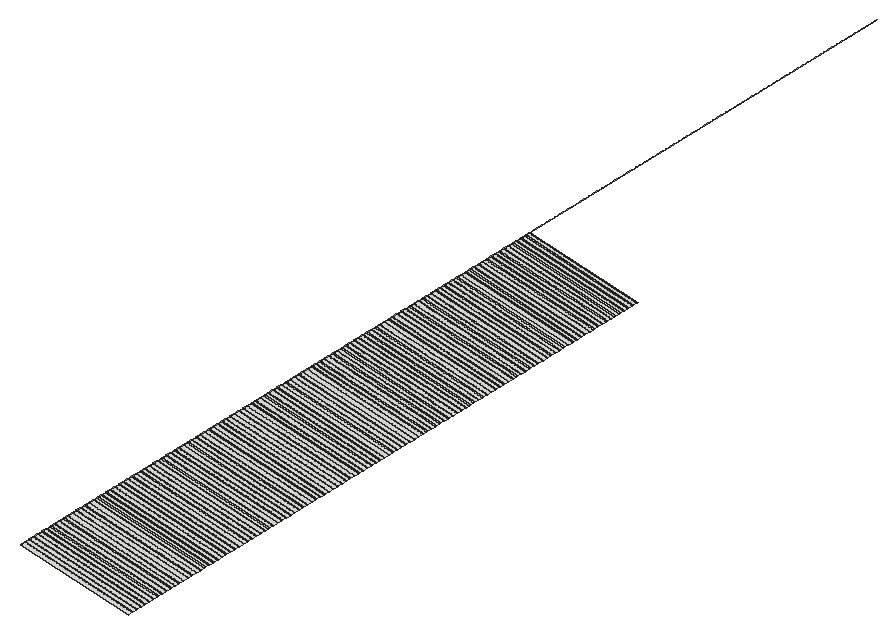
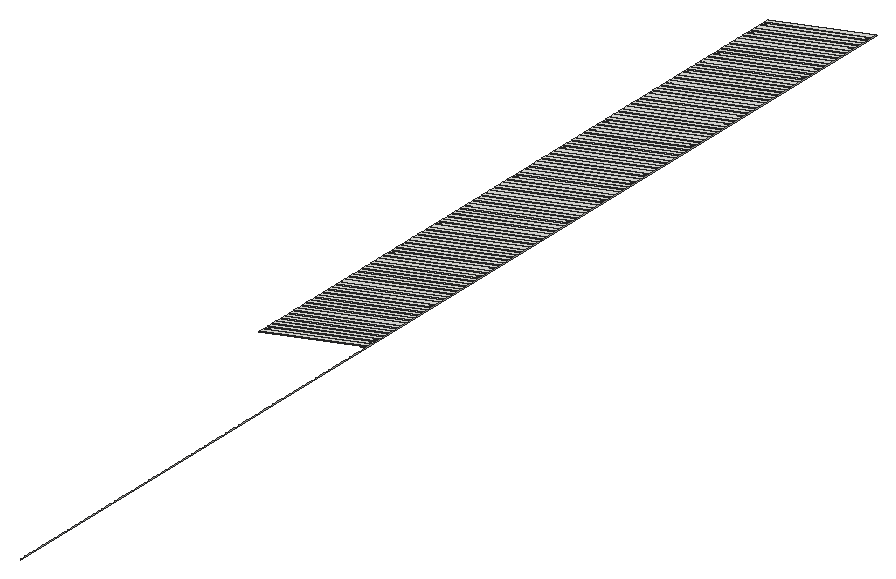
# SketchUp Ruby script. Lengths in inches.
U = 1.inch
M = Sketchup.active_model
def pt(a) = Geom::Point3d.new(a.map { |v| v * U })
def face(e, loops, mat)
  f = e.add_face(loops[0].map { |a| pt(a) })
  loops[1..].each { |l| e.add_face(l.map { |a| pt(a) }).erase! }
  f.material = f.back_material = mat if mat
  f
end
# faces: each face lists its corners as indices into pts; further lists are holes
def faces(e, pts, list, mat = nil) = list.each { |f| face(e, (f[0].is_a?(Array) ? f : [f]).map { |l| l.map { |i| pts[i] } }, mat) }
# xy, xz, yz: faces in a plane at the given z, y or x. An outline is a flat list of corners, or four numbers for a rectangle; further outlines are holes
def ring(l) = l.size == 4 ? [[l[0], l[1]], [l[2], l[1]], [l[2], l[3]], [l[0], l[3]]] : l.each_slice(2).to_a
def flat(e, list, mat, &to3) = list.each { |f| face(e, (f[0].is_a?(Array) ? f : [f]).map { |l| ring(l).map { |u, v| to3.(u, v) } }, mat) }
def xy(e, z, list, mat = nil) = flat(e, list, mat) { |x, y| [x, y, z] }
def xz(e, y, list, mat = nil) = flat(e, list, mat) { |x, z| [x, y, z] }
def yz(e, x, list, mat = nil) = flat(e, list, mat) { |y, z| [x, y, z] }
def lines(e, pts, list) = list.each { |a, b| e.add_line(pt(pts[a]), pt(pts[b])) }
# prism: a flat outline (further loops are holes) pulled along v
def prism(e, loops, v, mat = nil)
  f = face(e, loops, mat); d = Geom::Vector3d.new(v.map { |x| x * U })
  f.pushpull(f.normal.samedirection?(d) ? d.length : -d.length)
end
def box(e, o, s, mat = nil) = prism(e, [[o, [o[0] + s[0], o[1], o[2]], [o[0] + s[0], o[1] + s[1], o[2]], [o[0], o[1] + s[1], o[2]]]], [0, 0, s[2]], mat)
def at(x, y, z, deg = 0) = Geom::Transformation.translation(pt([x, y, z])) * Geom::Transformation.rotation(ORIGIN, Z_AXIS, deg.degrees)
def axes(o, x, y, z) = Geom::Transformation.new([*x, 0, *y, 0, *z, 0, *pt(o).to_a, 1])
def part(name) = M.definitions.add(name)
# library, detail: a bought-in or finely detailed component or shape, given as its bounding box
def library(name, o, s) = part(name).tap { |d| box(d.entities, o, s) }
def detail(e, o, s) = box(e.add_group.entities, o, s)
def put(e, d, t, mat = nil) = e.add_instance(d, t).tap { |i| i.material = mat if mat }
def group(e, t, mat = nil) = e.add_group.tap { |g| g.transformation = t; g.material = mat if mat }.entities
root = M.entities
p = [[2686.81,0,214.83],[2686.81,10.92,214.83],[2423.52,12.05,274.66],[2423.52,0,274.66],[2686.81,12.89,214.83],[2423.52,14.01,274.66],
  [2686.81,23.92,214.83],[2423.52,25.04,274.66],[2686.81,25.89,214.83],[2423.52,27.01,274.66],[2686.81,36.92,214.83],[2423.52,38.04,274.66],
  [2686.81,38.88,214.83],[2423.52,40.01,274.66],[2686.81,49.91,214.83],[2423.52,51.04,274.66],[2686.81,51.88,214.83],[2423.52,53.01,274.66],
  [2686.81,62.91,214.83],[2423.52,64.04,274.66],[2423.52,66,274.66],[2686.81,64.88,214.83],[2686.81,75.91,214.83],[2423.52,77.03,274.66],
  [2423.52,79,274.66],[2686.81,77.875,214.83],[2686.81,88.91,214.83],[2423.52,90.03,274.66],[2686.81,90.875,214.83],[2423.52,92,274.66],
  [2686.81,101.9,214.83],[2423.52,103.03,274.66],[2686.81,103.87,214.83],[2423.52,105,274.66],[2686.81,114.9,214.83],[2423.52,116.03,274.66],
  [2423.52,117.99,274.66],[2686.81,116.87,214.83],[2686.81,127.9,214.83],[2423.52,129.02,274.66],[2686.81,129.87,214.83],[2423.52,130.99,274.66],
  [2686.81,140.9,214.83],[2423.52,142.02,274.66],[2686.81,142.86,214.83],[2423.52,143.99,274.66],[2686.81,153.89,214.83],[2423.52,155.02,274.66],
  [2686.81,155.86,214.83],[2423.52,156.99,274.66],[2686.81,166.89,214.83],[2423.52,168.02,274.66],[2686.81,168.86,214.83],[2423.52,169.98,274.66],
  [2686.81,179.89,214.83],[2423.52,181.01,274.66],[2686.81,181.86,214.83],[2423.52,182.98,274.66],[2686.81,192.89,214.83],[2423.52,194.01,274.66],
  [2686.81,194.85,214.83],[2423.52,195.98,274.66],[2686.81,205.88,214.83],[2423.52,207.01,274.66],[2686.81,207.85,214.83],[2423.52,208.98,274.66],
  [2686.81,218.88,214.83],[2423.52,220.01,274.66],[2686.81,220.85,214.83],[2423.52,221.97,274.66],[2686.81,231.88,214.83],[2423.52,233,274.66],
  [2423.52,234.97,274.66],[2686.81,233.85,214.83],[2686.81,244.875,214.83],[2423.52,246,274.66],[2423.52,247.97,274.66],[2686.81,246.84,214.83],
  [2686.81,257.875,214.83],[2423.52,259,274.66],[2423.52,260.97,274.66],[2686.81,259.84,214.83],[2686.81,270.87,214.83],[2423.52,272,274.66],
  [2423.52,273.96,274.66],[2686.81,272.84,214.83],[2686.81,283.87,214.83],[2423.52,284.99,274.66],[2686.81,285.84,214.83],[2423.52,286.96,274.66],
  [2686.81,296.87,214.83],[2423.52,297.99,274.66],[2686.81,298.83,214.83],[2423.52,299.96,274.66],[2686.81,309.86,214.83],[2423.52,310.99,274.66],
  [2423.52,312.96,274.66],[2686.81,311.83,214.83],[2686.81,322.86,214.83],[2423.52,323.99,274.66],[2686.81,324.83,214.83],[2423.52,325.95,274.66],
  [2686.81,335.86,214.83],[2423.52,336.98,274.66],[2686.81,337.83,214.83],[2423.52,338.95,274.66],[2686.81,348.86,214.83],[2423.52,349.98,274.66],
  [2686.81,350.82,214.83],[2423.52,351.95,274.66],[2686.81,361.85,214.83],[2423.52,362.98,274.66],[2686.81,363.82,214.83],[2423.52,364.95,274.66],
  [2686.81,374.85,214.83],[2423.52,375.98,274.66],[2686.81,376.82,214.83],[2423.52,377.94,274.66],[2686.81,387.85,214.83],[2423.52,388.97,274.66],
  [2686.81,389.82,214.83],[2423.52,390.94,274.66],[2686.81,400.85,214.83],[2423.52,401.97,274.66],[2686.81,402.8125,214.83],[2423.52,403.9375,274.66],
  [2686.81,413.84,214.83],[2423.52,414.97,274.66],[2686.81,415.8125,214.83],[2423.52,416.9375,274.66],[2686.81,426.84,214.83],[2423.52,427.97,274.66],
  [2686.81,428.81,214.83],[2423.52,429.93,274.66],[2686.81,439.84,214.83],[2423.52,440.96,274.66],[2423.52,442.93,274.66],[2686.81,441.81,214.83],
  [2686.81,452.84,214.83],[2423.52,453.96,274.66],[2423.52,455.93,274.66],[2686.81,454.8,214.83],[2686.81,465.83,214.83],[2423.52,466.96,274.66],
  [2686.81,467.8,214.83],[2423.52,468.93,274.66],[2686.81,478.83,214.83],[2423.52,479.96,274.66],[2686.81,480.8,214.83],[2423.52,481.92,274.66],
  [2686.81,491.83,214.83],[2423.52,492.95,274.66],[2686.81,493.8,214.83],[2423.52,494.92,274.66],[2686.81,504.83,214.83],[2423.52,505.95,274.66],
  [2423.52,507.92,274.66],[2686.81,506.79,214.83],[2686.81,517.82,214.83],[2423.52,518.95,274.66],[2686.81,519.79,214.83],[2423.52,520.92,274.66],
  [2686.81,530.82,214.83],[2423.52,531.95,274.66],[2686.81,532.79,214.83],[2423.52,533.91,274.66],[2686.81,543.82,214.83],[2423.52,544.94,274.66],
  [2423.52,546.91,274.66],[2686.81,545.79,214.83],[2686.81,556.82,214.83],[2423.52,557.94,274.66],[2686.81,558.78,214.83],[2423.52,559.91,274.66],
  [2686.81,569.8125,214.83],[2423.52,570.9375,274.66],[2423.52,572.91,274.66],[2686.81,571.78,214.83],[2686.81,582.8125,214.83],[2423.52,583.9375,274.66],
  [2686.81,584.78,214.83],[2423.52,585.9,274.66],[2686.81,595.81,214.83],[2423.52,596.93,274.66],[2423.52,598.9,274.66],[2686.81,597.78,214.83],
  [2686.81,608.81,214.83],[2423.52,609.93,274.66],[2686.81,610.77,214.83],[2423.52,611.9,274.66],[2686.81,621.8,214.83],[2423.52,622.93,274.66],
  [2686.81,623.77,214.83],[2423.52,624.9,274.66],[2686.81,634.8,214.83],[2423.52,635.93,274.66],[2686.81,636.77,214.83],[2423.52,637.89,274.66],
  [2686.81,647.8,214.83],[2423.52,648.92,274.66],[2686.81,649.77,214.83],[2423.52,650.89,274.66],[2686.81,660.8,214.83],[2423.52,661.92,274.66],
  [2686.81,662.76,214.83],[2423.52,663.89,274.66],[2686.81,673.79,214.83],[2423.52,674.92,274.66],[2686.81,675.76,214.83],[2423.52,676.89,274.66],
  [2686.81,686.79,214.83],[2423.52,687.92,274.66],[2686.81,688.76,214.83],[2423.52,689.88,274.66],[2686.81,699.79,214.83],[2423.52,700.91,274.66],
  [2423.52,702.88,274.66],[2686.81,701.76,214.83],[2686.81,712.79,214.83],[2423.52,713.91,274.66],[2423.52,715.88,274.66],[2686.81,714.75,214.83],
  [2686.81,725.78,214.83],[2423.52,726.91,274.66],[2423.52,728.88,274.66],[2686.81,727.75,214.83],[2686.81,738.78,214.83],[2423.52,739.91,274.66],
  [2686.81,740.75,214.83],[2423.52,741.875,274.66],[2686.81,751.78,214.83],[2423.52,752.9,274.66],[2686.81,753.75,214.83],[2423.52,754.87,274.66],
  [2686.81,764.78,214.83],[2423.52,765.9,274.66],[2423.52,767.87,274.66],[2686.81,766.74,214.83],[2686.81,777.77,214.83],[2423.52,778.9,274.66],
  [2686.81,779.74,214.83],[2423.52,780.87,274.66],[2686.81,790.77,214.83],[2423.52,791.9,274.66],[2686.81,792.74,214.83],[2423.52,793.86,274.66],
  [2686.81,803.77,214.83],[2423.52,804.89,274.66],[2686.81,805.74,214.83],[2423.52,806.86,274.66],[2686.81,816.77,214.83],[2423.52,817.89,274.66],
  [2423.52,819.86,274.66],[2686.81,818.73,214.83],[2686.81,829.76,214.83],[2423.52,830.89,274.66],[2686.81,831.73,214.83],[2423.52,832.86,274.66],
  [2686.81,842.76,214.83],[2423.52,843.89,274.66],[2686.81,844.75,214.83],[2423.52,845.875,274.66],[2686.81,855.76,214.83],[2423.52,856.88,274.66],
  [2686.81,857.76,214.83],[2423.52,858.89,274.66],[2686.81,868.76,214.83],[2423.52,869.88,274.66],[2686.81,870.78,214.83],[2423.52,871.9,274.66],
  [2686.81,881.75,214.83],[2423.52,882.88,274.66],[2686.81,883.79,214.83],[2423.52,884.91,274.66],[2686.81,894.75,214.83],[2423.52,895.875,274.66],
  [2686.81,896.8,214.83],[2423.52,897.93,274.66],[2686.81,907.75,214.83],[2423.52,908.875,274.66],[2686.81,909.82,214.83],[2423.52,910.94,274.66],
  [2686.81,920.75,214.83],[2423.52,921.87,274.66],[2686.81,922.83,214.83],[2423.52,923.95,274.66],[2686.81,933.74,214.83],[2423.52,934.87,274.66],
  [2686.81,935.84,214.83],[2423.52,936.97,274.66],[2686.81,946.74,214.83],[2423.52,947.87,274.66],[2686.81,948.86,214.83],[2423.52,949.98,274.66],
  [2686.81,959.74,214.83],[2423.52,960.86,274.66],[2686.81,961.87,214.83],[2423.52,962.99,274.66],[2686.81,972.74,214.83],[2423.52,973.86,274.66],
  [2686.81,974.88,214.83],[2423.52,976.01,274.66],[2686.81,985.73,214.83],[2423.52,986.86,274.66],[2686.81,987.9,214.83],[2423.52,989.02,274.66],
  [2686.81,998.73,214.83],[2423.52,999.86,274.66],[2686.81,1000.91,214.83],[2423.52,1002.03,274.66],[2686.81,1011.73,214.83],[2423.52,1012.85,274.66],
  [2686.81,1013.92,214.83],[2423.52,1015.05,274.66],[2686.81,1024.73,214.83],[2423.52,1025.85,274.66],[2686.81,1026.9375,214.83],[2423.52,1028.0625,274.66],
  [2686.81,1037.72,214.83],[2423.52,1038.85,274.66],[2686.81,1039.95,214.83],[2423.52,1041.07,274.66],[2686.81,1050.72,214.83],[2423.52,1051.85,274.66],
  [2686.81,1052.96,214.83],[2423.52,1054.09,274.66],[2686.81,1063.72,214.83],[2423.52,1064.84,274.66],[2686.81,1065.98,214.83],[2423.52,1067.1,274.66],
  [2686.81,1076.72,214.83],[2423.52,1077.84,274.66],[2686.81,1078.99,214.83],[2423.52,1080.12,274.66],[2686.81,1089.71,214.83],[2423.52,1090.84,274.66],
  [2686.81,1092,214.83],[2423.52,1093.13,274.66],[2686.81,1102.71,214.83],[2423.52,1103.84,274.66],[2686.81,1105.02,214.83],[2423.52,1106.14,274.66],
  [2686.81,1115.71,214.83],[2423.52,1116.83,274.66],[2686.81,1118.03,214.83],[2423.52,1119.16,274.66],[2686.81,1128.71,214.83],[2423.52,1129.83,274.66],
  [2686.81,1131.04,214.83],[2423.52,1132.17,274.66],[2686.81,1141.7,214.83],[2423.52,1142.83,274.66],[2686.81,1144.06,214.83],[2423.52,1145.18,274.66],
  [2686.81,1154.7,214.83],[2423.52,1155.83,274.66],[2686.81,1157.07,214.83],[2423.52,1158.2,274.66],[2686.81,1167.7,214.83],[2423.52,1168.82,274.66],
  [2686.81,1170.08,214.83],[2423.52,1171.21,274.66],[2686.81,1180.7,214.83],[2423.52,1181.82,274.66],[2686.81,1183.1,214.83],[2423.52,1184.22,274.66],
  [2686.81,1193.69,214.83],[2423.52,1194.82,274.66],[2686.81,1196.11,214.83],[2423.52,1197.24,274.66],[2686.81,1206.69,214.83],[2423.52,1207.82,274.66],
  [2686.81,1209.125,214.83],[2423.52,1210.25,274.66],[2686.81,1219.69,214.83],[2423.52,1220.81,274.66],[2686.81,1222.14,214.83],[2423.52,1223.26,274.66],
  [2686.81,1232.6875,214.83],[2423.52,1233.8125,274.66],[2686.81,1235.15,214.83],[2423.52,1236.28,274.66],[2686.81,1245.68,214.83],[2423.52,1246.81,274.66],
  [2686.81,1248.16,214.83],[2423.52,1249.29,274.66],[2686.81,1258.68,214.83],[2423.52,1259.81,274.66],[2686.81,1261.18,214.83],[2423.52,1262.3,274.66],
  [2686.81,1271.68,214.83],[2423.52,1272.8,274.66],[2686.81,1274.19,214.83],[2423.52,1275.32,274.66],[2686.81,1284.68,214.83],[2423.52,1285.8,274.66],
  [2686.81,1287.21,214.83],[2423.52,1288.33,274.66],[2686.81,1297.67,214.83],[2423.52,1298.8,274.66],[2686.81,1300.22,214.83],[2423.52,1301.34,274.66],
  [2686.81,1310.67,214.83],[2423.52,1311.8,274.66],[2686.81,1313.23,214.83],[2423.52,1314.36,274.66],[2686.81,1323.67,214.83],[2423.52,1324.79,274.66],
  [2686.81,1326.25,214.83],[2423.52,1327.37,274.66],[2686.81,1336.67,214.83],[2423.52,1337.79,274.66],[2686.81,1339.26,214.83],[2423.52,1340.38,274.66],
  [2686.81,1349.66,214.83],[2423.52,1350.79,274.66],[2686.81,1352.27,214.83],[2423.52,1353.4,274.66],[2686.81,1362.66,214.83],[2423.52,1363.79,274.66],
  [2686.81,1365.29,214.83],[2423.52,1366.41,274.66],[2686.81,1375.66,214.83],[2423.52,1376.78,274.66],[2686.81,1378.3,214.83],[2423.52,1379.42,274.66],
  [2686.81,1388.66,214.83],[2423.52,1389.78,274.66],[2686.81,1391.3125,214.83],[2423.52,1392.4375,274.66],[2686.81,1401.65,214.83],[2423.52,1402.78,274.66],
  [2686.81,1404.33,214.83],[2423.52,1405.45,274.66],[2686.81,1414.65,214.83],[2423.52,1415.78,274.66],[2686.81,1417.34,214.83],[2423.52,1418.46,274.66],
  [2686.81,1427.65,214.83],[2423.52,1428.77,274.66],[2686.81,1430.35,214.83],[2423.52,1431.48,274.66],[2686.81,1440.65,214.83],[2423.52,1441.77,274.66],
  [2686.81,1443.37,214.83],[2423.52,1444.49,274.66],[2686.81,1453.65,214.83],[2423.52,1454.77,274.66],[2686.81,1456.38,214.83],[2423.52,1457.5,274.66],
  [2686.81,1466.64,214.83],[2423.52,1467.77,274.66],[2686.81,1469.39,214.83],[2423.52,1470.52,274.66],[2686.81,1479.64,214.83],[2423.52,1480.77,274.66],
  [2686.81,1482.41,214.83],[2423.52,1483.53,274.66],[2686.81,1492.64,214.83],[2423.52,1493.76,274.66],[2686.81,1495.42,214.83],[2423.52,1496.55,274.66],
  [2686.81,1505.64,214.83],[2423.52,1506.76,274.66],[2686.81,1507.6,214.83],[2423.52,1508.73,274.66],[2423.52,1509.56,274.66],[2686.81,1508.43,214.83],
  [2686.81,1518.63,214.83],[2423.52,1519.76,274.66],[2686.81,1520.6,214.83],[2423.52,1521.73,274.66],[2423.52,1522.57,274.66],[2686.81,1521.45,214.83],
  [2686.81,1531.63,214.83],[2423.52,1532.76,274.66],[2686.81,1533.6,214.83],[2423.52,1534.72,274.66],[2423.52,1535.59,274.66],[2686.81,1534.46,214.83],
  [2686.81,1544.63,214.83],[2423.52,1545.75,274.66],[2686.81,1546.6,214.83],[2423.52,1547.72,274.66],[2423.52,1548.6,274.66],[2686.81,1547.47,214.83],
  [2423.3,2602.6875,273.6875],[2423.3,0,273.6875],[2423.52,1558.75,274.66],[2423.52,1560.72,274.66],[2423.52,1561.61,274.66],[2423.52,1571.75,274.66],
  [2423.52,1573.72,274.66],[2423.52,1574.625,274.66],[2423.52,1584.75,274.66],[2423.52,1586.71,274.66],[2423.52,1587.64,274.66],[2423.52,1597.74,274.66],
  [2423.52,1599.71,274.66],[2423.52,1600.65,274.66],[2423.52,1610.74,274.66],[2423.52,1612.71,274.66],[2423.52,1613.67,274.66],[2423.52,1623.74,274.66],
  [2423.52,1625.71,274.66],[2423.52,1626.68,274.66],[2423.52,1636.74,274.66],[2423.52,1638.7,274.66],[2423.52,1639.69,274.66],[2423.52,1649.73,274.66],
  [2423.52,1651.7,274.66],[2423.52,1652.71,274.66],[2423.52,1662.73,274.66],[2423.52,1664.7,274.66],[2423.52,1665.72,274.66],[2423.52,1675.73,274.66],
  [2423.52,1677.7,274.66],[2423.52,1678.73,274.66],[2423.52,1688.73,274.66],[2423.52,1690.69,274.66],[2423.52,1691.75,274.66],[2423.52,1701.72,274.66],
  [2423.52,1703.69,274.66],[2423.52,1704.76,274.66],[2423.52,1714.72,274.66],[2423.52,1716.6875,274.66],[2423.52,1717.77,274.66],[2423.52,1727.72,274.66],
  [2423.52,1729.6875,274.66],[2423.52,1730.79,274.66],[2423.52,1740.72,274.66],[2423.52,1742.68,274.66],[2423.52,1743.8,274.66],[2423.52,1753.71,274.66],
  [2423.52,1755.68,274.66],[2423.52,1756.8125,274.66],[2423.52,1766.71,274.66],[2423.52,1768.68,274.66],[2423.52,1769.83,274.66],[2423.52,1779.71,274.66],
  [2423.52,1781.68,274.66],[2423.52,1782.84,274.66],[2423.52,1792.71,274.66],[2423.52,1794.67,274.66],[2423.52,1795.85,274.66],[2423.52,1805.7,274.66],
  [2423.52,1807.67,274.66],[2423.52,1808.87,274.66],[2423.52,1818.7,274.66],[2423.52,1820.67,274.66],[2423.52,1821.88,274.66],[2423.52,1831.7,274.66],
  [2423.52,1833.67,274.66],[2423.52,1834.89,274.66],[2423.52,1844.7,274.66],[2423.52,1846.66,274.66],[2423.52,1847.91,274.66],[2423.52,1857.69,274.66],
  [2423.52,1859.66,274.66],[2423.52,1860.92,274.66],[2423.52,1870.69,274.66],[2423.52,1872.66,274.66],[2423.52,1873.94,274.66],[2423.52,1883.6875,274.66],
  [2423.52,1885.66,274.66],[2423.52,1886.95,274.66],[2423.52,1896.6875,274.66],[2423.52,1898.65,274.66],[2423.52,1899.96,274.66],[2423.52,1909.68,274.66],
  [2423.52,1911.65,274.66],[2423.52,1912.98,274.66],[2423.52,1922.68,274.66],[2423.52,1924.65,274.66],[2423.52,1925.99,274.66],[2423.52,1935.68,274.66],
  [2423.52,1937.65,274.66],[2423.52,1939,274.66],[2423.52,1948.68,274.66],[2423.52,1950.64,274.66],[2423.52,1952.02,274.66],[2423.52,1961.67,274.66],
  [2423.52,1963.64,274.66],[2423.52,1965.03,274.66],[2423.52,1974.67,274.66],[2423.52,1976.64,274.66],[2423.52,1978.04,274.66],[2423.52,1987.67,274.66],
  [2423.52,1989.64,274.66],[2423.52,1991.06,274.66],[2423.52,2000.67,274.66],[2423.52,2002.63,274.66],[2423.52,2004.07,274.66],[2423.52,2013.66,274.66],
  [2423.52,2015.63,274.66],[2423.52,2017.08,274.66],[2423.52,2026.66,274.66],[2423.52,2028.63,274.66],[2423.52,2030.1,274.66],[2423.52,2039.66,274.66],
  [2423.52,2041.625,274.66],[2423.52,2043.11,274.66],[2423.52,2052.66,274.66],[2423.52,2054.625,274.66],[2423.52,2056.125,274.66],[2423.52,2065.65,274.66],
  [2423.52,2067.62,274.66],[2423.52,2069.14,274.66],[2423.52,2078.65,274.66],[2423.52,2080.62,274.66],[2423.52,2082.15,274.66],[2423.52,2091.65,274.66],
  [2423.52,2093.62,274.66],[2423.52,2095.16,274.66],[2423.52,2104.65,274.66],[2423.52,2106.61,274.66],[2423.52,2108.18,274.66],[2423.52,2117.64,274.66],
  [2423.52,2119.61,274.66],[2423.52,2121.19,274.66],[2423.52,2130.64,274.66],[2423.52,2132.61,274.66],[2423.52,2134.2,274.66],[2423.52,2143.64,274.66],
  [2423.52,2145.61,274.66],[2423.52,2147.22,274.66],[2423.52,2156.64,274.66],[2423.52,2158.6,274.66],[2423.52,2160.23,274.66],[2423.52,2169.63,274.66],
  [2423.52,2171.6,274.66],[2423.52,2173.24,274.66],[2423.52,2182.63,274.66],[2423.52,2184.6,274.66],[2423.52,2186.26,274.66],[2423.52,2195.63,274.66],
  [2423.52,2197.6,274.66],[2423.52,2199.27,274.66],[2423.52,2208.625,274.66],[2423.52,2210.59,274.66],[2423.52,2212.28,274.66],[2423.52,2221.625,274.66],
  [2423.52,2223.59,274.66],[2423.52,2225.3,274.66],[2423.52,2234.62,274.66],[2423.52,2236.59,274.66],[2423.52,2238.3125,274.66],[2423.52,2247.62,274.66],
  [2423.52,2249.59,274.66],[2423.52,2251.32,274.66],[2423.52,2260.62,274.66],[2423.52,2262.58,274.66],[2423.52,2264.34,274.66],[2423.52,2273.61,274.66],
  [2423.52,2275.58,274.66],[2423.52,2277.35,274.66],[2423.52,2286.61,274.66],[2423.52,2288.58,274.66],[2423.52,2290.37,274.66],[2423.52,2299.61,274.66],
  [2423.52,2301.58,274.66],[2423.52,2303.38,274.66],[2423.52,2312.61,274.66],[2423.52,2314.57,274.66],[2423.52,2316.39,274.66],[2423.52,2325.6,274.66],
  [2423.52,2327.57,274.66],[2423.52,2329.41,274.66],[2423.52,2338.6,274.66],[2423.52,2340.57,274.66],[2423.52,2342.42,274.66],[2423.52,2351.6,274.66],
  [2423.52,2353.57,274.66],[2423.52,2355.43,274.66],[2423.52,2364.6,274.66],[2423.52,2366.56,274.66],[2423.52,2368.45,274.66],[2423.52,2377.59,274.66],
  [2423.52,2379.5625,274.66],[2423.52,2381.46,274.66],[2423.52,2390.59,274.66],[2423.52,2392.56,274.66],[2423.52,2394.47,274.66],[2423.52,2403.59,274.66],
  [2423.52,2405.56,274.66],[2423.52,2407.49,274.66],[2423.52,2416.59,274.66],[2423.52,2418.55,274.66],[2423.52,2420.5,274.66],[2423.52,2429.58,274.66],
  [2423.52,2431.55,274.66],[2423.52,2433.51,274.66],[2423.52,2442.58,274.66],[2423.52,2444.55,274.66],[2423.52,2446.53,274.66],[2423.52,2455.58,274.66],
  [2423.52,2457.55,274.66],[2423.52,2459.54,274.66],[2423.52,2468.58,274.66],[2423.52,2470.54,274.66],[2423.52,2472.55,274.66],[2423.52,2481.57,274.66],
  [2423.52,2483.54,274.66],[2423.52,2485.57,274.66],[2423.52,2494.57,274.66],[2423.52,2496.54,274.66],[2423.52,2498.58,274.66],[2423.52,2507.57,274.66],
  [2423.52,2509.54,274.66],[2423.52,2511.59,274.66],[2423.52,2520.57,274.66],[2423.52,2522.53,274.66],[2423.52,2524.61,274.66],[2423.52,2533.5625,274.66],
  [2423.52,2535.53,274.66],[2423.52,2537.62,274.66],[2423.52,2546.5625,274.66],[2423.52,2548.53,274.66],[2423.52,2550.63,274.66],[2423.52,2559.56,274.66],
  [2423.52,2561.53,274.66],[2423.52,2563.65,274.66],[2423.52,2572.56,274.66],[2423.52,2574.52,274.66],[2423.52,2576.66,274.66],[2423.52,2585.55,274.66],
  [2423.52,2587.52,274.66],[2423.52,2589.67,274.66],[2423.52,2598.55,274.66],[2423.52,2600.52,274.66],[2423.52,2602.6875,274.66],[2417.45,0,275.02],
  [2686.81,-1.125,214.83]]
faces(root,p,[[0,1,2,3],[2,1,4,5],[4,6,7,5],[6,8,9,7],[8,10,11,9],[10,12,13,11],[12,14,15,13],[14,16,17,15],
  [16,18,19,17],[20,19,18,21],[21,22,23,20],[24,23,22,25],[25,26,27,24],[26,28,29,27],[28,30,31,29],[30,32,33,31],
  [32,34,35,33],[36,35,34,37],[37,38,39,36],[38,40,41,39],[40,42,43,41],[42,44,45,43],[44,46,47,45],[46,48,49,47],
  [48,50,51,49],[50,52,53,51],[52,54,55,53],[54,56,57,55],[56,58,59,57],[58,60,61,59],[60,62,63,61],[62,64,65,63],
  [64,66,67,65],[66,68,69,67],[68,70,71,69],[72,71,70,73],[73,74,75,72],[76,75,74,77],[77,78,79,76],[80,79,78,81],
  [81,82,83,80],[84,83,82,85],[85,86,87,84],[86,88,89,87],[88,90,91,89],[90,92,93,91],[92,94,95,93],[96,95,94,97],
  [97,98,99,96],[98,100,101,99],[100,102,103,101],[102,104,105,103],[104,106,107,105],[106,108,109,107],[108,110,111,109],[110,112,113,111],
  [112,114,115,113],[114,116,117,115],[116,118,119,117],[118,120,121,119],[120,122,123,121],[122,124,125,123],[124,126,127,125],[126,128,129,127],
  [128,130,131,129],[130,132,133,131],[132,134,135,133],[136,135,134,137],[137,138,139,136],[140,139,138,141],[141,142,143,140],[142,144,145,143],
  [144,146,147,145],[146,148,149,147],[148,150,151,149],[150,152,153,151],[152,154,155,153],[156,155,154,157],[157,158,159,156],[158,160,161,159],
  [160,162,163,161],[162,164,165,163],[164,166,167,165],[168,167,166,169],[169,170,171,168],[170,172,173,171],[172,174,175,173],[176,175,174,177],
  [177,178,179,176],[178,180,181,179],[180,182,183,181],[184,183,182,185],[185,186,187,184],[186,188,189,187],[188,190,191,189],[190,192,193,191],
  [192,194,195,193],[194,196,197,195],[196,198,199,197],[198,200,201,199],[200,202,203,201],[202,204,205,203],[204,206,207,205],[206,208,209,207],
  [208,210,211,209],[210,212,213,211],[212,214,215,213],[216,215,214,217],[217,218,219,216],[220,219,218,221],[221,222,223,220],[224,223,222,225],
  [225,226,227,224],[226,228,229,227],[228,230,231,229],[230,232,233,231],[232,234,235,233],[236,235,234,237],[237,238,239,236],[238,240,241,239],
  [240,242,243,241],[242,244,245,243],[244,246,247,245],[246,248,249,247],[248,250,251,249],[252,251,250,253],[253,254,255,252],[254,256,257,255],
  [256,258,259,257],[259,258,260,261],[260,262,263,261],[262,264,265,263],[264,266,267,265],[267,266,268,269],[268,270,271,269],[270,272,273,271],
  [272,274,275,273],[275,274,276,277],[276,278,279,277],[278,280,281,279],[280,282,283,281],[282,284,285,283],[284,286,287,285],[286,288,289,287],
  [288,290,291,289],[290,292,293,291],[292,294,295,293],[294,296,297,295],[296,298,299,297],[299,298,300,301],[300,302,303,301],[303,302,304,305],
  [304,306,307,305],[307,306,308,309],[308,310,311,309],[310,312,313,311],[312,314,315,313],[314,316,317,315],[316,318,319,317],[319,318,320,321],
  [320,322,323,321],[322,324,325,323],[324,326,327,325],[326,328,329,327],[328,330,331,329],[330,332,333,331],[332,334,335,333],[334,336,337,335],
  [336,338,339,337],[338,340,341,339],[340,342,343,341],[342,344,345,343],[344,346,347,345],[346,348,349,347],[348,350,351,349],[350,352,353,351],
  [352,354,355,353],[354,356,357,355],[356,358,359,357],[358,360,361,359],[360,362,363,361],[362,364,365,363],[364,366,367,365],[366,368,369,367],
  [368,370,371,369],[371,370,372,373],[372,374,375,373],[374,376,377,375],[376,378,379,377],[378,380,381,379],[380,382,383,381],[382,384,385,383],
  [384,386,387,385],[386,388,389,387],[388,390,391,389],[390,392,393,391],[392,394,395,393],[394,396,397,395],[396,398,399,397],[398,400,401,399],
  [400,402,403,401],[402,404,405,403],[404,406,407,405],[406,408,409,407],[408,410,411,409],[410,412,413,411],[412,414,415,413],[414,416,417,415],
  [416,418,419,417],[419,418,420,421],[420,422,423,421],[423,422,424,425],[424,426,427,425],[426,428,429,427],[428,430,431,429],[430,432,433,431],
  [432,434,435,433],[434,436,437,435],[436,438,439,437],[439,438,440,441],[440,442,443,441],[442,444,445,443],[444,446,447,445],[446,448,449,447],
  [448,450,451,449],[450,452,453,451],[452,454,455,453],[454,456,457,455],[456,458,459,457],[459,458,460,461],[460,462,463,461],[463,462,464,465],
  [466,465,464,467],[467,468,469,466],[469,468,470,471],[472,471,470,473],[473,474,475,472],[475,474,476,477],[478,477,476,479],[479,480,481,478],
  [481,480,482,483],[484,483,482,485],[486,487,3,2,5,7,9,11,13,15,17,19,20,23,24,27,29,31,33,35,36,39,41,43,45,47,49,51,53,55,57,59,61,63,65,67,69,71,72,75,76,79,80,83,84,87,89,91,93,95,96,99,101,103,105,107,109,111,113,115,117,119,121,123,125,127,129,131,133,135,136,139,140,143,145,147,149,151,153,155,156,159,161,163,165,167,168,171,173,175,176,179,181,183,184,187,189,191,193,195,197,199,201,203,205,207,209,211,213,215,216,219,220,223,224,227,229,231,233,235,236,239,241,243,245,247,249,251,252,255,257,259,261,263,265,267,269,271,273,275,277,279,281,283,285,287,289,291,293,295,297,299,301,303,305,307,309,311,313,315,317,319,321,323,325,327,329,331,333,335,337,339,341,343,345,347,349,351,353,355,357,359,361,363,365,367,369,371,373,375,377,379,381,383,385,387,389,391,393,395,397,399,401,403,405,407,409,411,413,415,417,419,421,423,425,427,429,431,433,435,437,439,441,443,445,447,449,451,453,455,457,459,461,463,465,466,469,471,472,475,477,478,481,483,484,488,489,490,491,492,493,494,495,496,497,498,499,500,501,502,503,504,505,506,507,508,509,510,511,512,513,514,515,516,517,518,519,520,521,522,523,524,525,526,527,528,529,530,531,532,533,534,535,536,537,538,539,540,541,542,543,544,545,546,547,548,549,550,551,552,553,554,555,556,557,558,559,560,561,562,563,564,565,566,567,568,569,570,571,572,573,574,575,576,577,578,579,580,581,582,583,584,585,586,587,588,589,590,591,592,593,594,595,596,597,598,599,600,601,602,603,604,605,606,607,608,609,610,611,612,613,614,615,616,617,618,619,620,621,622,623,624,625,626,627,628,629,630,631,632,633,634,635,636,637,638,639,640,641,642,643,644,645,646,647,648,649,650,651,652,653,654,655,656,657,658,659,660,661,662,663,664,665,666,667,668,669,670,671,672,673,674,675,676,677,678,679,680,681,682,683,684,685,686,687,688,689,690,691,692,693,694,695,696,697,698,699,700,701,702,703,704,705,706,707,708,709,710,711,712,713,714,715,716,717,718,719,720,721,722,723,724,725,726,727,728,729,730]])
lines(root,p,[[487,731],[732,3]])
